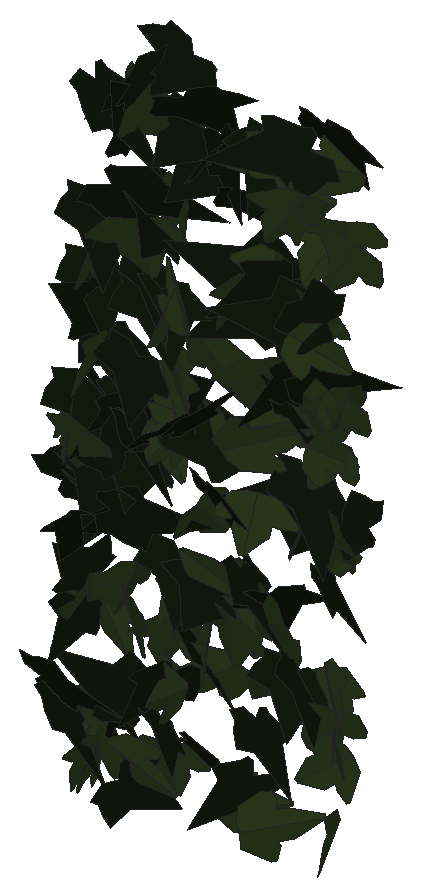
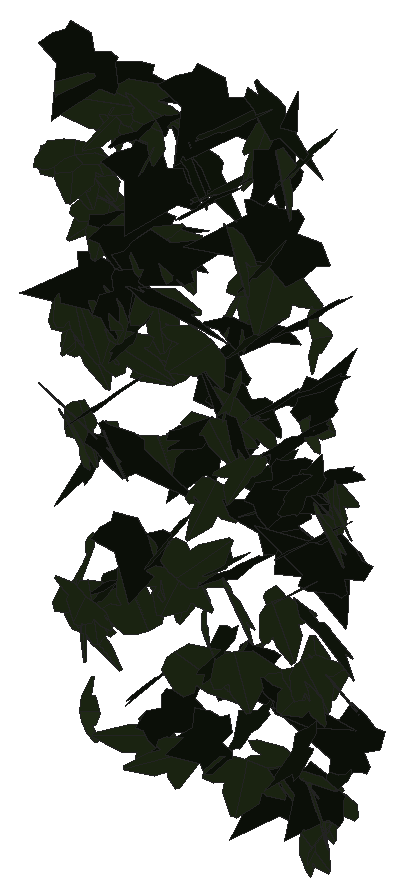
# SketchUp Ruby script. Lengths in inches.
U = 1.inch
M = Sketchup.active_model
def pt(a) = Geom::Point3d.new(a.map { |v| v * U })
def face(e, loops, mat)
  f = e.add_face(loops[0].map { |a| pt(a) })
  loops[1..].each { |l| e.add_face(l.map { |a| pt(a) }).erase! }
  f.material = f.back_material = mat if mat
  f
end
# faces: each face lists its corners as indices into pts; further lists are holes
def faces(e, pts, list, mat = nil) = list.each { |f| face(e, (f[0].is_a?(Array) ? f : [f]).map { |l| l.map { |i| pts[i] } }, mat) }
# xy, xz, yz: faces in a plane at the given z, y or x. An outline is a flat list of corners, or four numbers for a rectangle; further outlines are holes
def ring(l) = l.size == 4 ? [[l[0], l[1]], [l[2], l[1]], [l[2], l[3]], [l[0], l[3]]] : l.each_slice(2).to_a
def flat(e, list, mat, &to3) = list.each { |f| face(e, (f[0].is_a?(Array) ? f : [f]).map { |l| ring(l).map { |u, v| to3.(u, v) } }, mat) }
def xy(e, z, list, mat = nil) = flat(e, list, mat) { |x, y| [x, y, z] }
def xz(e, y, list, mat = nil) = flat(e, list, mat) { |x, z| [x, y, z] }
def yz(e, x, list, mat = nil) = flat(e, list, mat) { |y, z| [x, y, z] }
def lines(e, pts, list) = list.each { |a, b| e.add_line(pt(pts[a]), pt(pts[b])) }
# prism: a flat outline (further loops are holes) pulled along v
def prism(e, loops, v, mat = nil)
  f = face(e, loops, mat); d = Geom::Vector3d.new(v.map { |x| x * U })
  f.pushpull(f.normal.samedirection?(d) ? d.length : -d.length)
end
def box(e, o, s, mat = nil) = prism(e, [[o, [o[0] + s[0], o[1], o[2]], [o[0] + s[0], o[1] + s[1], o[2]], [o[0], o[1] + s[1], o[2]]]], [0, 0, s[2]], mat)
def at(x, y, z, deg = 0) = Geom::Transformation.translation(pt([x, y, z])) * Geom::Transformation.rotation(ORIGIN, Z_AXIS, deg.degrees)
def axes(o, x, y, z) = Geom::Transformation.new([*x, 0, *y, 0, *z, 0, *pt(o).to_a, 1])
def part(name) = M.definitions.add(name)
# library, detail: a bought-in or finely detailed component or shape, given as its bounding box
def library(name, o, s) = part(name).tap { |d| box(d.entities, o, s) }
def detail(e, o, s) = box(e.add_group.entities, o, s)
def put(e, d, t, mat = nil) = e.add_instance(d, t).tap { |i| i.material = mat if mat }
def group(e, t, mat = nil) = e.add_group.tap { |g| g.transformation = t; g.material = mat if mat }.entities
root = M.entities
M.materials.add("1026 AP 7946 SUNNY SIDE UP").color = [254, 231, 186]
M.materials.add("efeu1").color = [18, 25, 13]
M.materials.add("efeu2").color = [43, 57, 29]
c1 = part("ivyleaf_10")
p = [[0,0.5,-0.03],[-0.0625,2.02,-0.43],[-0.19,2.01,-0.46],[-0.54,1.05,-0.29],[-0.52,0.625,-0.18],[-0.83,0.76,-0.28],
  [-1.16,0.64,-0.33],[-1.15,0.33,-0.24],[-0.77,-0.39,0.02],[-0.3,-0.51,0.16],[0.04,-0.48,0.23],[-0.02,2.01,-0.4375],
  [-0.06,2.01,-0.43],[0.04,-0.49,0.23],[0.67,-0.49,0.14],[1.38,0.36,-0.2],[1.375,0.51,-0.24],[0.81,0.65,-0.19],
  [0.62,0.59,-0.15],[0.6,1.09,-0.28],[0.5,1.23,-0.31]]
faces(c1.entities,p,[[0,1,2,3,4,5,6,7,8,9,10],[11,12,0,13,14,15,16,17,18,19,20]],"efeu2")
c2 = part("ivyleaf_9")
p = [[1.54,2.16,1.25],[1.36,2.04,1.19],[-0.21,0.99,0.68],[-0.71,1.11,0.82],[-0.85,0.86,0.67],[-0.8,0.17,0.21],
  [-0.9,-0.01,0.1],[-0.67,-0.16,-0.02],[-0.08,-0.08,-0.05],[-0.03,-0.6,-0.4],[0.65,-0.88,-0.66],[0.83,-0.6,-0.49],
  [1.29,-0.42,-0.43],[1.8125,-0.07,-0.26],[1.21,0.44,0.15]]
faces(c2.entities,p,[[0,1,2,3,4,5,6,7,8,9,10,11,12,13,14]],"efeu1")
put(root,c1,axes([132.06,212.05,280.48],[0.20333,-0.29406,-0.08971],[-0.05456,0.07805,-0.33048],[0.4784,0.13389,0.00044]),"1026 AP 7946 SUNNY SIDE UP")
put(root,c1,axes([132.01,211.89,284.9],[0.35447,-0.24601,0.01411],[-0.00877,-0.02554,-0.34319],[0.38745,0.22449,-0.02067]),"1026 AP 7946 SUNNY SIDE UP")
put(root,c1,axes([131.87,211.74,285.12],[0.22296,-0.15991,0.26489],[0.2547,-0.20101,-0.22121],[0.40369,0.21514,-0.00674]),"1026 AP 7946 SUNNY SIDE UP")
put(root,c1,axes([132.05,212.18,279.8125],[0.04104,-0.27267,0.1874],[0.07433,-0.17901,-0.28206],[0.51139,0.0479,0.02596]),"1026 AP 7946 SUNNY SIDE UP")
put(root,c2,axes([132.16,211.99,286.7],[0.02564,0.05569,0.37929],[-0.35692,-0.29025,0.05393],[0.46351,-0.22658,0.02055]),"1026 AP 7946 SUNNY SIDE UP")
put(root,c2,axes([131.95,211.97,280.6],[0.48291,-0.02515,-0.08777],[-0.13677,-0.02543,-0.31596],[0.02729,0.31766,-0.03037]),"1026 AP 7946 SUNNY SIDE UP")
put(root,c1,axes([131.97,212.15,279.71],[-0.11776,-0.04133,0.33129],[0.24472,-0.29438,-0.00336],[0.44766,0.15005,0.08899]),"1026 AP 7946 SUNNY SIDE UP")
put(root,c1,axes([131.84,211.92,280.57],[0.42088,0.0219,0.17794],[0.27067,0.0127,-0.27659],[-0.03976,0.31824,0.00067]),"1026 AP 7946 SUNNY SIDE UP")
put(root,c2,axes([132.41,211.49,282.93],[-0.09843,0.26937,0.2029],[-0.16465,0.17281,-0.27893],[-0.49671,-0.11066,0.05225]),"1026 AP 7946 SUNNY SIDE UP")
put(root,c1,axes([132.21,212.01,282.45],[-0.14682,-0.29284,0.12332],[-0.00136,-0.12629,-0.31534],[0.49844,-0.08661,0.03546]),"1026 AP 7946 SUNNY SIDE UP")
put(root,c2,axes([132,212.22,287.21],[-0.04407,-0.34791,0.00492],[0.00688,-0.00712,-0.35958],[0.54711,-0.02793,0.00492]),"1026 AP 7946 SUNNY SIDE UP")
put(root,c2,axes([131.88,211.5,280.78],[0.31892,-0.33576,-0.03105],[-0.05185,0.01302,-0.40343],[0.52727,0.20437,-0.02089]),"1026 AP 7946 SUNNY SIDE UP")
put(root,c2,axes([132.23,211.66,282.31],[-0.42477,0.04293,-0.17547],[0.24961,-0.07511,-0.27892],[-0.1191,-0.31053,0.04125]),"1026 AP 7946 SUNNY SIDE UP")
put(root,c2,axes([131.73,211.42,281.09],[0.27396,-0.12668,0.27242],[0.34137,-0.15226,-0.22279],[0.31141,0.27836,0.00456]),"1026 AP 7946 SUNNY SIDE UP")
put(root,c1,axes([132.18,211.86,282.15],[-0.19948,-0.33019,-0.0532],[-0.04774,-0.04161,0.3639],[-0.52288,0.12977,-0.01293]),"1026 AP 7946 SUNNY SIDE UP")
put(root,c2,axes([131.82,211.77,284.05],[0.0752,-0.0057,0.34449],[0.50419,-0.09534,-0.04947],[0.14964,0.32409,-0.00644]),"1026 AP 7946 SUNNY SIDE UP")
put(root,c1,axes([132.44,211.39,285.09],[-0.47914,0.03581,0.14296],[-0.22064,-0.01055,-0.31513],[-0.04432,-0.33458,0.02326]),"1026 AP 7946 SUNNY SIDE UP")
put(root,c2,axes([132.22,212.17,283.87],[-0.17077,-0.26804,0.1793],[-0.02059,-0.18151,-0.29488],[0.5034,-0.09835,0.04876]),"1026 AP 7946 SUNNY SIDE UP")
put(root,c1,axes([132.25,211.85,287.82],[-0.11103,0.14997,-0.33504],[-0.02616,-0.33334,-0.15617],[-0.56374,-0.01407,0.07324]),"1026 AP 7946 SUNNY SIDE UP")
put(root,c1,axes([132.36,211.65,280.16],[0.00885,-0.32606,0.10618],[0.01847,-0.10469,-0.33643],[0.53828,0.00895,0.00979]),"1026 AP 7946 SUNNY SIDE UP")
put(root,c2,axes([132.19,211.85,285.57],[-0.14666,-0.33361,-0.09271],[0.05678,0.08132,-0.35616],[0.53958,-0.09924,0.01228]),"1026 AP 7946 SUNNY SIDE UP")
put(root,c1,axes([132.31,211.82,280.43],[0.35814,-0.24808,0.05614],[0.03221,-0.0569,-0.34646],[0.39856,0.22751,-0.02244]),"1026 AP 7946 SUNNY SIDE UP")
put(root,c2,axes([132.19,212.05,288.25],[-0.05961,-0.37513,0.06634],[0.00058,-0.06689,-0.38875],[0.59906,-0.03726,0.00698]),"1026 AP 7946 SUNNY SIDE UP")
put(root,c1,axes([132.29,212.07,282.14],[-0.44225,0.04162,-0.15597],[0.19603,-0.13037,-0.27584],[-0.15069,-0.29173,0.09893]),"1026 AP 7946 SUNNY SIDE UP")
put(root,c2,axes([132.15,212.17,285.43],[0.11464,-0.25044,0.22888],[0.10913,-0.21262,-0.2699],[0.5165,0.10051,0.00623]),"1026 AP 7946 SUNNY SIDE UP")
put(root,c2,axes([132.38,211.88,284.43],[-0.16228,-0.31284,0.14978],[-0.02126,-0.14981,-0.33873],[0.5432,-0.09932,0.03149]),"1026 AP 7946 SUNNY SIDE UP")
put(root,c2,axes([132.31,212.11,286.3],[0.05355,-0.33631,-0.08781],[-0.00464,0.08345,-0.34771],[0.54479,0.03377,0.00567]),"1026 AP 7946 SUNNY SIDE UP")
put(root,c1,axes([132.46,211.68,286.35],[0.10876,-0.20917,0.2878],[0.1172,-0.27062,-0.22836],[0.53763,0.10131,-0.00844]),"1026 AP 7946 SUNNY SIDE UP")
put(root,c2,axes([132.68,211.23,284.02],[0.06692,0.33494,-0.17567],[-0.0278,-0.17156,-0.34881],[-0.5917,0.04594,-0.00348]),"1026 AP 7946 SUNNY SIDE UP")
put(root,c2,axes([132.39,211.83,281.08],[0.35659,-0.22591,-0.10863],[-0.14472,0.05475,-0.32844],[0.3634,0.24348,-0.02421]),"1026 AP 7946 SUNNY SIDE UP")
put(root,c2,axes([132.76,212.08,285.39],[-0.07652,0.06432,-0.37699],[0.13308,-0.35782,-0.0784],[-0.56945,-0.09227,0.03234]),"1026 AP 7946 SUNNY SIDE UP")
put(root,c2,axes([133.05,211.46,285.1],[-0.47649,0.04437,-0.21927],[-0.3233,0.06153,0.31478],[0.11233,0.36531,-0.02415]),"1026 AP 7946 SUNNY SIDE UP")
put(root,c1,axes([132.77,211.91,290.47],[0.15096,-0.33609,-0.08634],[-0.0098,0.0833,-0.35921],[0.54385,0.09479,0.01749]),"1026 AP 7946 SUNNY SIDE UP")
put(root,c2,axes([132.55,211.56,290.54],[0.33208,-0.34965,-0.1623],[-0.08466,0.14876,-0.4189],[0.59576,0.21603,0.03094]),"1026 AP 7946 SUNNY SIDE UP")
put(root,c2,axes([133.29,211.35,281.3],[-0.17884,0.10542,0.32993],[-0.40903,0.1866,-0.15765],[-0.33588,-0.28337,0.01632]),"1026 AP 7946 SUNNY SIDE UP")
put(root,c1,axes([132.94,211.78,283.02],[-0.13812,-0.33159,0.06324],[-0.00629,-0.06435,-0.35353],[0.53076,-0.08705,0.01227]),"1026 AP 7946 SUNNY SIDE UP")
put(root,c2,axes([133.01,211.78,289.96],[0.10912,0.17604,0.44313],[-0.34606,-0.36947,0.19064],[0.64203,-0.22907,0.02744]),"1026 AP 7946 SUNNY SIDE UP")
put(root,c2,axes([132.9375,211.9,284.84],[-0.18612,-0.30357,0.10571],[0.06679,-0.12504,-0.32588],[0.50031,-0.09624,0.08283]),"1026 AP 7946 SUNNY SIDE UP")
put(root,c1,axes([133.07,211.75,288.4],[-0.49982,-0.22239,-0.07136],[0.10918,0.01916,-0.3988],[0.34899,-0.3245,0.02256]),"1026 AP 7946 SUNNY SIDE UP")
put(root,c2,axes([133.13,211.33,280.01],[0.02942,-0.03918,-0.38091],[-0.16947,0.35352,-0.04217],[0.55919,0.1092,0.00726]),"1026 AP 7946 SUNNY SIDE UP")
put(root,c2,axes([133.09,211.72,286.375],[-0.09304,-0.32535,0.11618],[-0.0138,-0.11483,-0.34115],[0.54223,-0.05875,0.01125]),"1026 AP 7946 SUNNY SIDE UP")
put(root,c2,axes([133.49,211.45,291.07],[-0.4016,0.27671,-0.11609],[0.09286,-0.10067,-0.38775],[-0.46149,-0.26106,0.02301]),"1026 AP 7946 SUNNY SIDE UP")
put(root,c2,axes([133,211.73,285.29],[0.23089,-0.30602,0.04566],[0.01128,-0.0476,-0.34965],[0.48647,0.14634,-0.01356]),"1026 AP 7946 SUNNY SIDE UP")
put(root,c2,axes([132.9,211.5,289.11],[0.08082,0.09113,-0.40705],[0.26375,0.3584,0.1096],[0.58136,-0.17527,0.00687]),"1026 AP 7946 SUNNY SIDE UP")
put(root,c2,axes([133.1,212.04,287.62],[0.02186,-0.33427,0.11278],[0.02899,-0.11061,-0.34504],[0.55326,0.019,0.01363]),"1026 AP 7946 SUNNY SIDE UP")
put(root,c1,axes([133.41,212.11,282.19],[-0.27477,-0.28345,0.04832],[-0.01587,-0.05069,-0.34284],[0.4519,-0.17413,0.01734]),"1026 AP 7946 SUNNY SIDE UP")
put(root,c1,axes([133.27,211.33,282.84],[-0.30928,0.27067,-0.07682],[0.04551,-0.07289,-0.34456],[-0.43975,-0.1979,0.01836]),"1026 AP 7946 SUNNY SIDE UP")
put(root,c1,axes([133.05,211.44,280.39],[-0.29991,0.0078,-0.28652],[0.42789,-0.06532,-0.19449],[-0.09153,-0.3309,0.02963]),"1026 AP 7946 SUNNY SIDE UP")
put(root,c2,axes([133.25,211.95,288.53],[-0.08662,-0.22295,0.29247],[-0.01623,-0.28736,-0.23519],[0.56894,-0.04214,0.03782]),"1026 AP 7946 SUNNY SIDE UP")
put(root,c1,axes([133.36,211.54,290.56],[-0.07298,-0.33418,-0.20485],[0.16074,0.1808,-0.33981],[0.58836,-0.09085,0.06743]),"1026 AP 7946 SUNNY SIDE UP")
put(root,c1,axes([133.46,211.92,280.35],[-0.51128,-0.09258,-0.02583],[0.05073,-0.02405,-0.34688],[0.1418,-0.3252,0.03094]),"1026 AP 7946 SUNNY SIDE UP")
put(root,c2,axes([133.07,211.26,284.22],[0.2971,0.05787,-0.28077],[0.24995,0.24849,0.16914],[0.36042,-0.22003,0.11415]),"1026 AP 7946 SUNNY SIDE UP")
put(root,c1,axes([133.59,211.96,288.98],[0.365,-0.23164,-0.13975],[-0.08255,0.13497,-0.33242],[0.41289,0.23176,0.05708]),"1026 AP 7946 SUNNY SIDE UP")
put(root,c2,axes([133.52,212.35,290.97],[-0.27906,-0.22574,0.22517],[-0.03208,-0.24356,-0.27603],[0.49443,-0.14321,0.10918]),"1026 AP 7946 SUNNY SIDE UP")
put(root,c1,axes([133.43,211.81,285.33],[0.09356,0.34152,0.09057],[0.03732,0.08311,-0.35652],[-0.5525,0.06345,-0.00875]),"1026 AP 7946 SUNNY SIDE UP")
put(root,c2,axes([133.49,211.76,287.54],[-0.2753,-0.25286,-0.15724],[0.19382,0.09687,-0.31338],[0.42076,-0.21007,0.04148]),"1026 AP 7946 SUNNY SIDE UP")
put(root,c2,axes([133.62,212.33,289.91],[-0.28512,-0.23183,0.22932],[-0.0333,-0.2478,-0.28341],[0.5057,-0.14702,0.11063]),"1026 AP 7946 SUNNY SIDE UP")
put(root,c1,axes([133.36,211.91,286.125],[0.48127,-0.04267,0.22413],[0.33015,-0.06458,-0.31737],[0.11311,0.37006,-0.02729]),"1026 AP 7946 SUNNY SIDE UP")
put(root,c1,axes([133.7,211.85,283.07],[0.35418,-0.25586,0.00324],[-0.01796,-0.01618,-0.35071],[0.40197,0.22471,-0.01853]),"1026 AP 7946 SUNNY SIDE UP")
put(root,c2,axes([133.48,211.74,280.93],[0.06058,-0.26639,0.20095],[0.03671,-0.19522,-0.2784],[0.51928,0.04488,-0.00376]),"1026 AP 7946 SUNNY SIDE UP")
put(root,c2,axes([133.85,211.53,281.85],[-0.01973,0.17277,-0.3008],[0.04458,-0.29161,-0.18012],[-0.53293,-0.03079,-0.00393]),"1026 AP 7946 SUNNY SIDE UP")
put(root,c1,axes([133.68,211.85,286.47],[-0.11871,0.32907,-0.03899],[0.00249,-0.04038,-0.34797],[-0.52119,-0.07515,0.00722]),"1026 AP 7946 SUNNY SIDE UP")
put(root,c2,axes([133.52,212.03,285.73],[-0.03093,0.14248,0.33918],[0.14343,-0.31608,0.14504],[0.54435,0.09138,-0.01895]),"1026 AP 7946 SUNNY SIDE UP")
put(root,c1,axes([133.77,211.54,287.43],[-0.05915,0.05912,-0.37701],[-0.00628,-0.36821,-0.06295],[-0.58338,-0.00203,0.0389]),"1026 AP 7946 SUNNY SIDE UP")
put(root,c1,axes([133.8,211.63,285.53],[-0.18005,-0.01885,0.34772],[0.17573,-0.33854,0.0176],[0.50184,0.11178,0.11859]),"1026 AP 7946 SUNNY SIDE UP")
put(root,c2,axes([133.79,211.79,283.47],[-0.12391,-0.32754,0.06327],[0.00064,-0.06511,-0.34708],[0.52454,-0.0773,0.01537]),"1026 AP 7946 SUNNY SIDE UP")
put(root,c2,axes([133.96,211.14,285.85],[0.12477,0.32812,0.06887],[0.03692,0.06117,-0.34731],[-0.52466,0.08233,-0.00806]),"1026 AP 7946 SUNNY SIDE UP")
put(root,c1,axes([134.04,211.44,287.46],[-0.08793,0.31616,-0.19703],[-0.09534,0.18479,0.33095],[0.57463,0.07904,0.02476]),"1026 AP 7946 SUNNY SIDE UP")
put(root,c2,axes([133.97,212.28,289.54],[-0.23599,-0.2356,0.25328],[-0.1165,-0.24112,-0.2845],[0.52416,-0.15966,0.0508]),"1026 AP 7946 SUNNY SIDE UP")
put(root,c1,axes([133.97,211.91,285.79],[0.5342,-0.01051,-0.067],[-0.10226,-0.00082,-0.35016],[0.01598,0.34589,-0.00084]),"1026 AP 7946 SUNNY SIDE UP")
put(root,c1,axes([133.93,211.51,281.61],[-0.06606,0.07843,0.35767],[0.15256,-0.33337,0.08784],[0.53778,0.10421,0.01902]),"1026 AP 7946 SUNNY SIDE UP")
put(root,c1,axes([134.35,212.05,281.86],[-0.29308,-0.12595,0.29622],[-0.30716,-0.21628,-0.22875],[0.3877,-0.26656,0.0427]),"1026 AP 7946 SUNNY SIDE UP")
put(root,c2,axes([133.81,211.96,282.2],[0.32065,-0.26218,0.00474],[-0.02335,-0.01925,-0.34143],[0.4117,0.2031,-0.02306]),"1026 AP 7946 SUNNY SIDE UP")
put(root,c2,axes([134.32,211.84,289.97],[-0.29816,0.26358,-0.15967],[0.13048,-0.133,-0.33515],[-0.464,-0.20678,0.00836]),"1026 AP 7946 SUNNY SIDE UP")
put(root,c1,axes([134.48,211.93,283.3],[-0.27091,-0.15239,-0.25411],[-0.33633,-0.12542,0.23383],[-0.30606,0.27271,-0.03203]),"1026 AP 7946 SUNNY SIDE UP")
put(root,c2,axes([134.52,211.96,285.42],[-0.26937,-0.0331,0.32196],[-0.38323,-0.21105,-0.16179],[0.31245,-0.28739,0.07913]),"1026 AP 7946 SUNNY SIDE UP")
put(root,c2,axes([134.13,211.49,290.89],[0.43464,0.2767,0.04104],[0.0749,0.00636,-0.40177],[-0.43279,0.27898,-0.02831]),"1026 AP 7946 SUNNY SIDE UP")
put(root,c1,axes([134.24,211.66,284.5],[-0.15266,-0.25825,-0.23622],[0.13394,0.21135,-0.28296],[0.52468,-0.12909,0.0035]),"1026 AP 7946 SUNNY SIDE UP")
put(root,c1,axes([134.12,211.9375,282.375],[0.2314,-0.20133,0.21695],[0.21788,-0.16063,-0.2575],[0.40447,0.20171,0.01459]),"1026 AP 7946 SUNNY SIDE UP")
put(root,c2,axes([133.97,211.84,280.62],[0.42279,-0.1448,0.08719],[0.11442,-0.04509,-0.31484],[0.23834,0.27851,-0.00353]),"1026 AP 7946 SUNNY SIDE UP")
put(root,c2,axes([134.29,211.79,283.23],[-0.2241,-0.23983,0.20346],[0.01596,-0.22214,-0.26979],[0.48962,-0.10253,0.10192]),"1026 AP 7946 SUNNY SIDE UP")
put(root,c1,axes([134.3,211.82,286.92],[-0.4652,0.06955,-0.19792],[0.27038,-0.0991,-0.3097],[-0.17459,-0.33877,0.04773]),"1026 AP 7946 SUNNY SIDE UP")
put(root,c2,axes([134.32,211.12,286.01],[0.1584,0.3554,0.01595],[-0.02944,-0.00867,0.38017],[0.55846,-0.10126,0.01552]),"1026 AP 7946 SUNNY SIDE UP")
put(root,c2,axes([134.3,212.03,290.07],[-0.16377,-0.01743,-0.36656],[0.55401,-0.05914,-0.10364],[-0.08174,-0.36591,0.03201]),"1026 AP 7946 SUNNY SIDE UP")
put(root,c2,axes([134.99,212.125,287.66],[-0.53644,0.01287,0.05635],[-0.08752,-0.03433,-0.34995],[-0.01134,-0.34379,0.03502]),"1026 AP 7946 SUNNY SIDE UP")
put(root,c2,axes([135.07,212.08,288.07],[-0.10026,0.03688,0.42882],[-0.6162,-0.15087,-0.04897],[0.2272,-0.39293,0.0564]),"1026 AP 7946 SUNNY SIDE UP")
put(root,c2,axes([134.62,211.375,285.05],[0.47907,-0.07968,-0.14988],[-0.22862,0.0162,-0.32373],[0.12424,0.33704,-0.01779]),"1026 AP 7946 SUNNY SIDE UP")
put(root,c1,axes([134.69,211.9,283],[-0.48654,-0.05474,-0.08081],[0.14104,-0.07658,-0.31111],[0.0511,-0.30981,0.0892]),"1026 AP 7946 SUNNY SIDE UP")
put(root,c1,axes([134.85,211.6,282.92],[-0.50107,0.10602,0.04594],[-0.0811,-0.01628,-0.34455],[-0.16125,-0.32127,0.03054]),"1026 AP 7946 SUNNY SIDE UP")
put(root,c1,axes([134.96,211.68,288.23],[-0.01951,-0.33484,0.1255],[-0.00821,-0.12362,-0.34591],[0.56124,-0.01345,-0.0007]),"1026 AP 7946 SUNNY SIDE UP")
put(root,c1,axes([134.74,211.74,280.1],[-0.04184,-0.0768,-0.34657],[0.35949,0.24823,-0.07565],[0.40551,-0.22797,0.03131]),"1026 AP 7946 SUNNY SIDE UP")
put(root,c2,axes([134.84,211.84,283.64],[0.2487,-0.31563,-0.07638],[-0.08571,0.05341,-0.36252],[0.5019,0.16552,-0.02406]),"1026 AP 7946 SUNNY SIDE UP")
put(root,c2,axes([134.97,211.83,289.57],[0.43426,0.22992,-0.01989],[0.00226,-0.03385,-0.36936],[-0.36297,0.27487,-0.02609]),"1026 AP 7946 SUNNY SIDE UP")
put(root,c2,axes([135.15,211.6,280.65],[-0.02058,0.01114,-0.36512],[0.13267,-0.34444,-0.01637],[-0.54166,-0.08479,0.00987]),"1026 AP 7946 SUNNY SIDE UP")
put(root,c1,axes([135.1,212.05,288.42],[-0.15513,-0.24127,0.25875],[0.11247,-0.27081,-0.23934],[0.53755,-0.01297,0.12475]),"1026 AP 7946 SUNNY SIDE UP")
put(root,c2,axes([135.03,211.89,281.35],[0.14566,-0.31802,-0.07273],[-0.03716,0.06477,-0.34083],[0.51028,0.0955,-0.00406]),"1026 AP 7946 SUNNY SIDE UP")
put(root,c1,axes([135.6,211.66,283.18],[-0.29885,0.10677,0.30164],[-0.43707,0.09547,-0.22164],[-0.21965,-0.33524,0.03063]),"1026 AP 7946 SUNNY SIDE UP")
put(root,c1,axes([135.35,211.5,287.14],[-0.27638,-0.29788,0.00685],[0.01288,-0.01451,-0.35609],[0.4684,-0.17537,0.01384]),"1026 AP 7946 SUNNY SIDE UP")
put(root,c2,axes([135.25,212.04,290.23],[-0.19744,-0.32221,0.11815],[-0.05448,-0.11152,-0.35681],[0.53599,-0.13002,0.00726]),"1026 AP 7946 SUNNY SIDE UP")
put(root,c1,axes([135.25,211.56,284.9375],[0.4141,0.19239,-0.06804],[-0.05262,-0.06739,-0.33456],[-0.31606,0.26329,-0.03345]),"1026 AP 7946 SUNNY SIDE UP")
put(root,c1,axes([135.25,211.73,289.88],[-0.16573,0.3308,-0.096],[0.0355,-0.09256,-0.35815],[-0.54004,-0.1076,0.00591]),"1026 AP 7946 SUNNY SIDE UP")
put(root,c2,axes([135.35,211.8,283.48],[0.2837,0.27117,-0.05007],[-0.01483,-0.05382,-0.33511],[-0.43336,0.17936,-0.02131]),"1026 AP 7946 SUNNY SIDE UP")
put(root,c1,axes([135.71,211.69,290.43],[0.24541,0.00901,-0.33553],[-0.50699,-0.04806,-0.1608],[-0.07424,0.35799,-0.01101]),"1026 AP 7946 SUNNY SIDE UP")
put(root,c1,axes([135.1,211.97,290.28],[-0.21706,0.07379,-0.34946],[0.31977,-0.27921,-0.14928],[-0.44319,-0.2376,0.06345]),"1026 AP 7946 SUNNY SIDE UP")
put(root,c2,axes([135.61,211.86,288.43],[-0.00399,0.04081,-0.37275],[-0.11781,-0.35439,-0.04268],[-0.56066,0.07418,0.01162]),"1026 AP 7946 SUNNY SIDE UP")
put(root,c2,axes([135.83,211.98,284.95],[-0.09789,-0.06347,-0.38324],[-0.53537,-0.15233,0.08466],[-0.25463,0.34466,-0.03068]),"1026 AP 7946 SUNNY SIDE UP")
put(root,c1,axes([135.45,211.77,282.11],[-0.15054,-0.35572,0.05352],[0.00784,0.05453,0.3797],[-0.56568,0.09542,-0.00898]),"1026 AP 7946 SUNNY SIDE UP")
put(root,c1,axes([135.86,211.82,286.4],[-0.26994,-0.03856,0.30545],[-0.37545,-0.18851,-0.16866],[0.28354,-0.28632,0.06748]),"1026 AP 7946 SUNNY SIDE UP")
put(root,c1,axes([135.32,211.18,286.01],[-0.17953,-0.15213,0.3398],[0.30319,0.2687,0.19749],[-0.48549,0.22406,-0.00232]),"1026 AP 7946 SUNNY SIDE UP")
put(root,c1,axes([135.38,211.42,280.04],[0.06123,0.00697,-0.40438],[0.42812,0.28375,0.03467],[0.44481,-0.27406,0.02229]),"1026 AP 7946 SUNNY SIDE UP")
put(root,c2,axes([136.05,211.68,290.67],[-0.06272,-0.11404,-0.35839],[-0.26433,-0.30443,0.12111],[-0.51029,0.17172,-0.01869]),"1026 AP 7946 SUNNY SIDE UP")
put(root,c2,axes([135.54,211.79,286.74],[0.27369,-0.30788,0.00062],[-0.01214,-0.00707,-0.36425],[0.48397,0.17393,-0.00949]),"1026 AP 7946 SUNNY SIDE UP")
put(root,c2,axes([136.19,211.54,288.06],[-0.29091,-0.00836,0.31358],[-0.45881,-0.09717,-0.186],[0.13718,-0.34274,0.04292]),"1026 AP 7946 SUNNY SIDE UP")
put(root,c2,axes([135.94,211.7,287.2],[-0.12454,0.04547,-0.36605],[0.19667,-0.33777,-0.07518],[-0.52824,-0.13648,0.05831]),"1026 AP 7946 SUNNY SIDE UP")
put(root,c1,axes([135.83,211.95,284.9],[0.24804,-0.28188,0.11288],[0.07494,-0.1007,-0.33328],[0.47053,0.16463,-0.00643]),"1026 AP 7946 SUNNY SIDE UP")
put(root,c1,axes([136.15,211.38,290.03],[-0.32047,-0.24567,0.15592],[-0.13379,-0.12768,-0.32926],[0.43476,-0.22039,0.01361]),"1026 AP 7946 SUNNY SIDE UP")
put(root,c2,axes([135.88,211.62,282.52],[-0.13438,-0.31087,0.03218],[0.00229,-0.03461,-0.33217],[0.49156,-0.08482,0.01035]),"1026 AP 7946 SUNNY SIDE UP")
put(root,c1,axes([136.42,212.0625,290.34],[-0.02148,0.0357,0.37333],[-0.39011,-0.26609,0.01582],[0.41868,-0.24609,0.03389]),"1026 AP 7946 SUNNY SIDE UP")
put(root,c1,axes([136.06,211.45,289.92],[0.06175,-0.13604,-0.36801],[0.1745,0.34692,-0.12177],[0.57398,-0.09083,0.07661]),"1026 AP 7946 SUNNY SIDE UP")
put(root,c1,axes([136.31,212,289.25],[-0.40624,-0.163,0.19197],[-0.06259,-0.23958,-0.2728],[0.38533,-0.21076,0.15807]),"1026 AP 7946 SUNNY SIDE UP")
put(root,c2,axes([135.98,211.71,282.43],[0.05811,-0.30953,0.16413],[0.01618,-0.16094,-0.32198],[0.54842,0.03755,-0.00789]),"1026 AP 7946 SUNNY SIDE UP")
put(root,c1,axes([136.23,211.62,288.32],[-0.52642,0.12187,-0.01299],[0.00112,-0.03676,-0.36555],[-0.19277,-0.33303,0.03336]),"1026 AP 7946 SUNNY SIDE UP")
put(root,c1,axes([136.03,211.71,286.92],[-0.34491,0.11676,-0.25214],[0.26391,-0.18985,-0.24871],[-0.33611,-0.26888,0.06346]),"1026 AP 7946 SUNNY SIDE UP")
put(root,c1,axes([136.45,211.9,286.78],[-0.49973,-0.0153,0.13631],[-0.20074,-0.06345,-0.32361],[0.06023,-0.33839,0.05246]),"1026 AP 7946 SUNNY SIDE UP")
put(root,c2,axes([136.07,211.81,285.44],[-0.00702,-0.42688,0.07563],[-0.00319,-0.07582,-0.44023],[0.68173,-0.00475,-0.00128]),"1026 AP 7946 SUNNY SIDE UP")
put(root,c1,axes([136.51,211.7,286.18],[-0.47721,0.10158,0.10876],[-0.21226,-0.10245,-0.30047],[-0.08781,-0.30436,0.13526]),"1026 AP 7946 SUNNY SIDE UP")
put(root,c2,axes([136.7,211.25,288.44],[-0.36843,0.22324,0.1445],[-0.17909,0.08165,-0.33242],[-0.37271,-0.25991,0.01689]),"1026 AP 7946 SUNNY SIDE UP")
put(root,c2,axes([136.0625,211.58,287.21],[0.07777,0.15304,-0.3371],[0.12324,0.31875,0.16722],[0.55575,-0.0921,0.01009]),"1026 AP 7946 SUNNY SIDE UP")
put(root,c1,axes([136.15,212.14,282.28],[0.43835,-0.05385,0.1604],[0.23428,-0.04958,-0.29221],[0.1116,0.31559,-0.01659]),"1026 AP 7946 SUNNY SIDE UP")
put(root,c1,axes([136.5,211.62,282.05],[-0.46002,-0.18515,0.04725],[-0.03796,-0.04928,-0.35576],[0.29792,-0.29217,0.02762]),"1026 AP 7946 SUNNY SIDE UP")
put(root,c2,axes([136.27,211.86,291.04],[0.56153,0.00486,-0.14025],[-0.21338,-0.02155,-0.36757],[-0.0192,0.38159,-0.01674]),"1026 AP 7946 SUNNY SIDE UP")
put(root,c1,axes([136.46,212.03,289.42],[-0.45497,-0.2119,-0.01824],[0.046,-0.0121,-0.36849],[0.33102,-0.28956,0.02614]),"1026 AP 7946 SUNNY SIDE UP")
put(root,c1,axes([136.7,211.6,284.9],[-0.32256,0.13936,0.22883],[-0.33238,0.07731,-0.25153],[-0.24219,-0.2917,0.04044]),"1026 AP 7946 SUNNY SIDE UP")
put(root,c1,axes([136.68,211.875,289.22],[-0.51683,-0.00088,0.14694],[-0.21798,-0.08241,-0.3301],[0.05282,-0.3487,0.07548]),"1026 AP 7946 SUNNY SIDE UP")
put(root,c1,axes([136.55,211.9,286.94],[-0.16759,-0.32483,0.05577],[-0.01173,-0.05644,-0.35236],[0.51817,-0.10634,0.01006]),"1026 AP 7946 SUNNY SIDE UP")
put(root,c1,axes([136.66,211.58,281.66],[-0.2418,0.25772,0.11749],[-0.18984,0.05539,-0.3002],[-0.39939,-0.18236,0.07156]),"1026 AP 7946 SUNNY SIDE UP")
put(root,c1,axes([136.77,211.49,281.54],[0.40842,-0.16288,-0.20765],[-0.29297,0.07911,-0.31418],[0.2816,0.31853,-0.02569]),"1026 AP 7946 SUNNY SIDE UP")
put(root,c1,axes([136.43,211.77,280.22],[0.11484,-0.132,0.31834],[0.23676,-0.2707,-0.157],[0.47356,0.16735,0.00129]),"1026 AP 7946 SUNNY SIDE UP")
put(root,c1,axes([136.56,211.74,284.48],[0.37382,-0.23261,0.11569],[-0.08078,0.10881,0.34085],[-0.39896,-0.23998,0.03939]),"1026 AP 7946 SUNNY SIDE UP")
put(root,c2,axes([136.44,211.52,284.33],[0.36281,-0.21624,-0.17301],[-0.20277,0.10608,-0.32501],[0.37843,0.26416,-0.00828]),"1026 AP 7946 SUNNY SIDE UP")
put(root,c1,axes([136.54,211.61,282.7],[-0.14442,0.32842,-0.08132],[0.02043,-0.08024,-0.35167],[-0.53142,-0.09234,0.00858]),"1026 AP 7946 SUNNY SIDE UP")
put(root,c2,axes([137.02,211.75,285.12],[-0.38012,0.20955,0.09348],[-0.12796,0.04255,-0.32866],[-0.33469,-0.25426,0.01949]),"1026 AP 7946 SUNNY SIDE UP")
put(root,c1,axes([136.5,211.06,288.11],[0.16613,0.19678,0.28282],[0.12914,0.26285,-0.22605],[-0.5137,0.12972,0.03463]),"1026 AP 7946 SUNNY SIDE UP")
put(root,c1,axes([136.62,211.26,286.37],[0.09211,0.18477,0.3078],[-0.01472,0.30258,-0.18978],[-0.55079,0.02281,0.05655]),"1026 AP 7946 SUNNY SIDE UP")
